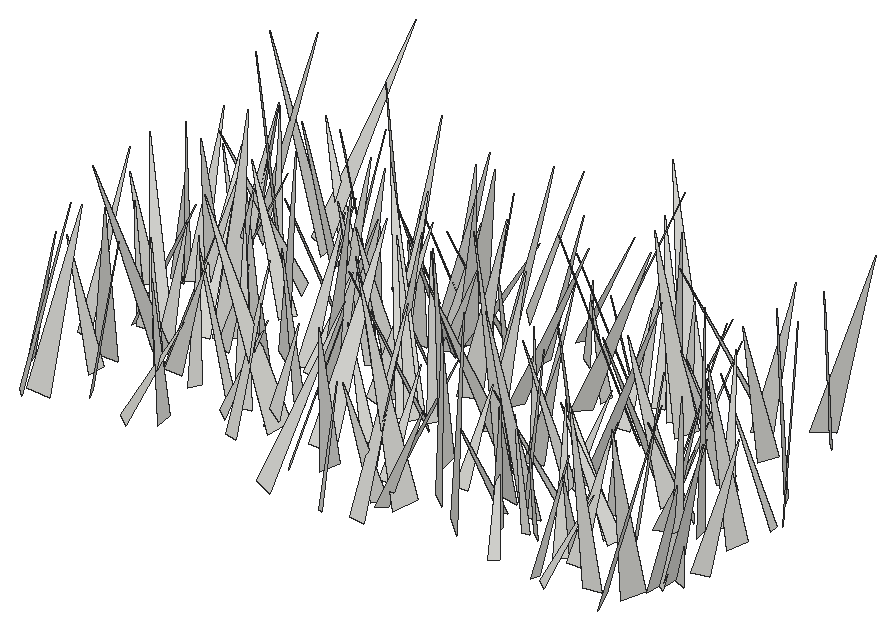
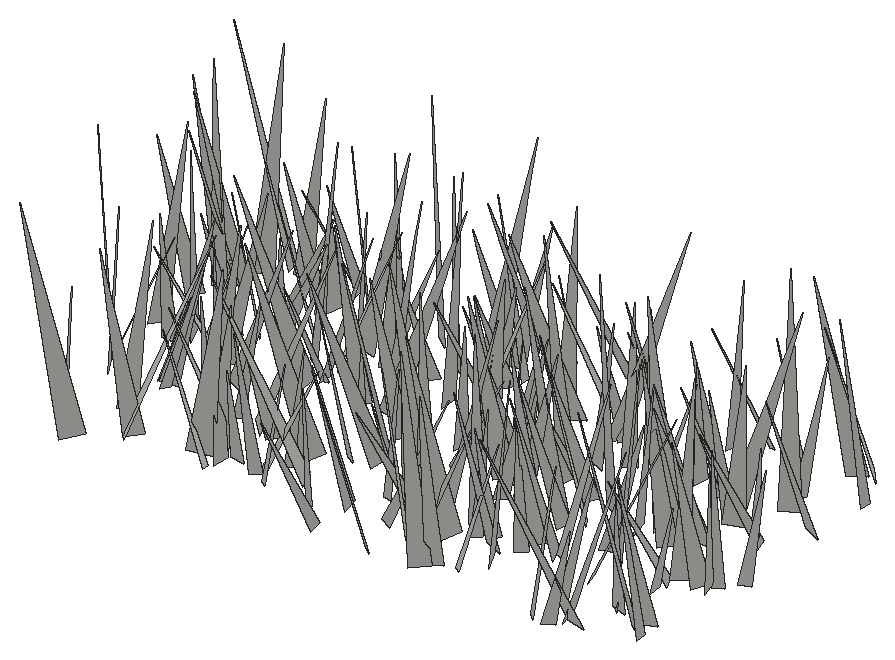
# SketchUp Ruby script. Lengths in inches.
U = 1.inch
M = Sketchup.active_model
def pt(a) = Geom::Point3d.new(a.map { |v| v * U })
def face(e, loops, mat)
  f = e.add_face(loops[0].map { |a| pt(a) })
  loops[1..].each { |l| e.add_face(l.map { |a| pt(a) }).erase! }
  f.material = f.back_material = mat if mat
  f
end
# faces: each face lists its corners as indices into pts; further lists are holes
def faces(e, pts, list, mat = nil) = list.each { |f| face(e, (f[0].is_a?(Array) ? f : [f]).map { |l| l.map { |i| pts[i] } }, mat) }
# xy, xz, yz: faces in a plane at the given z, y or x. An outline is a flat list of corners, or four numbers for a rectangle; further outlines are holes
def ring(l) = l.size == 4 ? [[l[0], l[1]], [l[2], l[1]], [l[2], l[3]], [l[0], l[3]]] : l.each_slice(2).to_a
def flat(e, list, mat, &to3) = list.each { |f| face(e, (f[0].is_a?(Array) ? f : [f]).map { |l| ring(l).map { |u, v| to3.(u, v) } }, mat) }
def xy(e, z, list, mat = nil) = flat(e, list, mat) { |x, y| [x, y, z] }
def xz(e, y, list, mat = nil) = flat(e, list, mat) { |x, z| [x, y, z] }
def yz(e, x, list, mat = nil) = flat(e, list, mat) { |y, z| [x, y, z] }
def lines(e, pts, list) = list.each { |a, b| e.add_line(pt(pts[a]), pt(pts[b])) }
# prism: a flat outline (further loops are holes) pulled along v
def prism(e, loops, v, mat = nil)
  f = face(e, loops, mat); d = Geom::Vector3d.new(v.map { |x| x * U })
  f.pushpull(f.normal.samedirection?(d) ? d.length : -d.length)
end
def box(e, o, s, mat = nil) = prism(e, [[o, [o[0] + s[0], o[1], o[2]], [o[0] + s[0], o[1] + s[1], o[2]], [o[0], o[1] + s[1], o[2]]]], [0, 0, s[2]], mat)
def at(x, y, z, deg = 0) = Geom::Transformation.translation(pt([x, y, z])) * Geom::Transformation.rotation(ORIGIN, Z_AXIS, deg.degrees)
def axes(o, x, y, z) = Geom::Transformation.new([*x, 0, *y, 0, *z, 0, *pt(o).to_a, 1])
def part(name) = M.definitions.add(name)
# library, detail: a bought-in or finely detailed component or shape, given as its bounding box
def library(name, o, s) = part(name).tap { |d| box(d.entities, o, s) }
def detail(e, o, s) = box(e.add_group.entities, o, s)
def put(e, d, t, mat = nil) = e.add_instance(d, t).tap { |i| i.material = mat if mat }
def group(e, t, mat = nil) = e.add_group.tap { |g| g.transformation = t; g.material = mat if mat }.entities
root = M.entities
c1 = part("fur_instance\#9")
p = [[0.8125,0,1.79],[0.67,-0.02,1.48],[0,-0.11,0],[0,0.11,0]]
faces(c1.entities,p,[[0,1,2,3]])
put(root,c1,axes([502.27,435.3,-21.66],[-0.87926,6.56228,2.62812],[6.83144,1.46959,-1.38397],[1.81713,-2.34956,6.47466]))
put(root,c1,axes([525.14,434.54,-21.66],[2.28996,3.33239,0.84649],[3.03653,-2.43723,1.38011],[-1.61271,0.14282,3.80053]))
put(root,c1,axes([546.94,438.2,-21.66],[6.05759,-4.04132,1.47541],[-3.82561,-6.22554,-1.34569],[-1.96821,-0.33746,7.15653]))
put(root,c1,axes([545.92,436.44,-21.66],[7.78659,2.72532,1.24866],[2.87625,-7.77148,-0.97412],[-0.84485,-1.33952,8.19204]))
put(root,c1,axes([508.52,435.88,-21.66],[2.58495,3.56171,0.23056],[3.43761,-2.40789,-1.34382],[0.96012,-0.96809,4.1907]))
put(root,c1,axes([527.24,437.77,-21.66],[2.70621,-3.86796,1.26709],[-3.69816,-2.97221,-1.17466],[-1.70008,0.30833,4.57219]))
put(root,c1,axes([510.52,437.41,-21.66],[5.22033,-0.21574,2.13038],[0.1303,-5.5713,-0.88347],[-2.13731,-0.86658,5.14955]))
put(root,c1,axes([501.4,434.64,-21.66],[4.49985,4.45709,1.03745],[4.28289,-4.6143,1.2473],[-1.61209,0.1822,6.20956]))
put(root,c1,axes([541.65,435.8,-21.66],[1.90499,3.12749,0.05078],[3.06447,-1.8542,-0.76405],[0.62675,-0.43991,3.5814]))
put(root,c1,axes([520.53,434.68,-21.66],[1.99959,6.47326,0.24716],[6.43471,-1.95494,-0.85747],[0.74746,-0.48749,6.72058]))
put(root,c1,axes([544.51,437.19,-21.66],[-0.07394,-6.12578,2.47714],[-6.56947,-0.19789,-0.68546],[-0.70961,2.47033,6.08776]))
put(root,c1,axes([499.51,437.95,-21.66],[5.83398,1.13984,1.03884],[1.35175,-5.73614,-1.2974],[-0.74243,-1.48703,5.80098]))
put(root,c1,axes([527.8,437.32,-21.66],[3.87779,-2.1954,0.31482],[-2.2129,-3.78759,0.8446],[0.14815,0.88911,4.37535]))
put(root,c1,axes([540.71,436.34,-21.66],[4.041,0.55824,1.1889],[0.26805,-4.11576,1.02147],[-1.28579,0.89645,3.94942]))
put(root,c1,axes([532.84,438.14,-21.66],[-4.52397,-6.09316,3.51067],[-6.34353,5.33763,1.08955],[3.03497,2.07386,7.51038]))
put(root,c1,axes([522.19,439.15,-21.66],[5.38586,-3.00561,1.16634],[-2.8404,-5.49795,-1.05176],[-1.52519,-0.37466,6.07741]))
put(root,c1,axes([528.85,438.31,-21.66],[-7.80525,1.8691,2.4402],[2.24771,8.01322,1.05174],[2.09664,-1.63243,7.95672]))
put(root,c1,axes([537.33,436.47,-21.66],[-3.18847,2.06393,0.29466],[1.98964,3.17316,-0.69666],[0.62286,0.42918,3.73374]))
put(root,c1,axes([527.66,435.03,-21.66],[1.84381,6.83005,0.32521],[6.75707,-1.87158,0.99709],[-1.04756,-0.05069,7.00393]))
put(root,c1,axes([525.7,438.75,-21.66],[5.69454,1.71793,1.14191],[1.95584,-5.5622,-1.38552],[-0.6557,-1.67144,5.78441]))
put(root,c1,axes([535.42,439.12,-21.66],[5.69502,0.05498,1.49404],[0.36012,-5.7612,-1.16071],[-1.45103,-1.21405,5.57575]))
put(root,c1,axes([504.93,437.25,-21.66],[4.32331,2.64676,1.47041],[2.57631,-4.56233,0.63737],[-1.59061,-0.19566,5.02892]))
put(root,c1,axes([540.91,440.02,-21.66],[3.64038,-1.44849,0.64201],[-1.22649,-3.59476,-1.15586],[-1.003,-0.8615,3.74359]))
put(root,c1,axes([503.36,439.67,-21.66],[-4.62696,1.13691,1.70574],[1.48296,4.76376,0.84751],[1.41525,-1.27471,4.68861]))
put(root,c1,axes([502.73,441.37,-21.66],[1.80193,-7.44469,0.50754],[-7.36471,-1.69029,1.35351],[1.20089,0.80465,7.53912]))
put(root,c1,axes([520.26,437.6,-21.66],[4.1336,3.03674,0.5342],[2.87698,-4.11997,1.15876],[-1.10914,0.6308,4.99657]))
put(root,c1,axes([541.75,438.98,-21.66],[-1.54169,4.36128,2.00643],[4.43238,2.10262,-1.16464],[1.84406,-1.40768,4.47674]))
put(root,c1,axes([537.59,440.31,-21.66],[-1.86728,-3.21645,1.13397],[-3.16749,2.11482,0.78275],[1.26429,0.54787,3.63587]))
put(root,c1,axes([530.01,440.18,-21.66],[-3.26006,-5.04679,2.60885],[-5.29814,3.78652,0.70434],[2.05082,1.75965,5.96674]))
put(root,c1,axes([547.6875,441.08,-21.66],[6.64533,-1.36705,0.39109],[-1.31179,-6.61549,-0.83466],[-0.54862,-0.74069,6.73295]))
put(root,c1,axes([534.12,441.43,-21.66],[-0.56318,-3.80765,0.20803],[-3.75255,0.51599,-0.71463],[-0.67806,0.30692,3.78215]))
put(root,c1,axes([515.02,438.35,-21.66],[1.99951,5.4557,0.6063],[5.41529,-2.06607,0.73224],[-0.89823,-0.31139,5.76424]))
put(root,c1,axes([516.68,441.11,-21.66],[-8.04315,1.60644,1.39343],[1.83623,7.99603,1.38066],[1.07265,-1.64234,8.08496]))
put(root,c1,axes([547.78,441.375,-21.66],[-1.4348,-7.0433,2.45033],[-7.23254,1.92235,1.29061],[1.81726,2.08982,7.07114]))
put(root,c1,axes([512.89,440.21,-21.66],[2.48404,3.35431,0.63876],[3.34518,-2.23213,-1.28736],[0.685,-1.26336,3.97047]))
put(root,c1,axes([527.1,439.61,-21.66],[-1.4583,4.1794,0.64732],[4.14586,1.27741,1.09233],[-0.83566,-0.95598,4.28962]))
put(root,c1,axes([540.46,439.14,-21.66],[-4.55116,2.07867,0.64916],[1.93391,4.54938,-1.00919],[1.00113,0.66152,4.90056]))
put(root,c1,axes([547.33,439.67,-21.66],[6.67173,1.075,1.66778],[0.88806,-6.84957,0.86244],[-1.77439,0.61387,6.70252]))
put(root,c1,axes([536.15,440.92,-21.66],[-4.08433,-4.26667,3.28401],[-4.58243,4.91876,0.69141],[2.82675,1.80893,5.86585]))
put(root,c1,axes([536.89,440.19,-21.66],[0.66208,3.60921,1.19442],[3.54519,-1.02396,1.12897],[-1.37285,-0.90361,3.49144]))
put(root,c1,axes([533.46,442.82,-21.66],[0.2783,-5.0487,0.14304],[-4.93686,-0.24166,1.07529],[1.0664,0.19877,4.94071]))
put(root,c1,axes([547.35,440.32,-21.66],[2.91311,4.64162,1.0633],[4.76072,-2.81168,-0.76908],[0.10392,-1.30816,5.4258]))
put(root,c1,axes([516.2,440.87,-21.66],[-1.839,3.01934,1.93742],[3.07994,2.44517,-0.88715],[1.83955,-1.07548,3.42218]))
put(root,c1,axes([526.01,439.94,-21.66],[-2.24412,3.20659,0.81725],[3.00578,2.38826,-1.11699],[1.38398,0.01256,3.75108]))
put(root,c1,axes([535.91,441.9375,-21.66],[-0.62718,-6.98929,2.39617],[-7.29856,0.2117,-1.29283],[-1.15016,2.46782,6.89725]))
put(root,c1,axes([513.98,443.21,-21.66],[1.58205,-4.94043,0.08132],[-4.90313,-1.55912,0.66773],[0.6114,0.28046,5.1444]))
put(root,c1,axes([507.17,442.52,-21.66],[2.31038,-4.41979,0.71264],[-4.3801,-2.06578,1.38834],[0.92579,1.25629,4.79008]))
put(root,c1,axes([505.16,443.98,-21.66],[-0.75565,-7.24529,1.23648],[-7.25287,0.53359,-1.30585],[-1.19119,1.34729,7.16659]))
put(root,c1,axes([541.84,442.8,-21.66],[-4.37284,2.10544,0.41102],[2.13916,4.20984,1.19366],[-0.16073,-1.25217,4.70423]))
put(root,c1,axes([513.35,441.64,-21.66],[-0.65155,5.99766,1.58433],[6.18323,0.49957,0.65163],[-0.49968,-1.63861,5.99765]))
put(root,c1,axes([509.35,441.95,-21.66],[-4.59387,1.36569,1.34916],[1.20913,4.77619,-0.71765],[1.49109,0.33451,4.73854]))
put(root,c1,axes([535.74,444.74,-21.66],[-3.80651,-3.12707,0.03174],[-3.06593,3.74155,0.93273],[0.61617,-0.70095,4.83716]))
put(root,c1,axes([538.64,443.25,-21.66],[3.81482,2.67004,0.71919],[2.75746,-3.58156,-1.32965],[0.20681,-1.49748,4.4625]))
put(root,c1,axes([530.23,442.125,-21.66],[-1.29453,3.3269,0.92168],[3.25121,1.50588,-0.8692],[1.16077,-0.50757,3.46245]))
put(root,c1,axes([548.49,442.92,-21.66],[3.34726,-4.07819,1.53745],[-4.35777,-3.09938,1.26621],[0.07255,1.99042,5.12177]))
put(root,c1,axes([520.33,440.74,-21.66],[-1.86477,7.56726,1.18834],[7.49142,2.05683,-1.34204],[1.5982,-0.81177,7.67722]))
put(root,c1,axes([511.8,442.32,-21.66],[-4.83845,-0.36416,0.05457],[-0.36621,4.6838,-1.21411],[-0.03844,1.21473,4.69778]))
put(root,c1,axes([527.66,443.93,-21.66],[-7.27615,-1.41209,3.18772],[-1.2687,7.94356,0.62294],[3.24745,-0.06052,7.38568]))
put(root,c1,axes([505.96,442.62,-21.66],[0.1057,3.9764,0.92499],[3.9126,-0.36287,1.11284],[-1.16573,-0.85739,3.81897]))
put(root,c1,axes([541.29,443.12,-21.66],[-3.62089,2.64212,0.01483],[2.58278,3.53416,0.96476],[-0.55698,-0.78788,4.37731]))
put(root,c1,axes([522.07,443.17,-21.66],[-2.23276,3.13779,0.67741],[3.20125,2.1153,0.75324],[-0.23799,-0.9847,3.77672]))
put(root,c1,axes([537.34,445.16,-21.66],[-4.05006,-5.82532,2.03849],[-5.82326,4.4146,1.04584],[2.04438,1.03428,7.01738]))
put(root,c1,axes([525.23,442.81,-21.66],[4.11341,0.99659,0.14821],[0.94897,-4.04143,0.83763],[-0.33855,0.78037,4.1487]))
put(root,c1,axes([506.24,442.92,-21.66],[4.19181,1.99584,0.5753],[1.88629,-4.2003,0.82769],[-0.86965,0.50967,4.56832]))
put(root,c1,axes([515.68,444.32,-21.66],[-1.40726,-4.75955,2.034],[-5.17479,1.24906,-0.65748],[-0.10975,2.13481,4.91949]))
put(root,c1,axes([539.56,445.42,-21.66],[0.99148,-3.49866,0.36174],[-3.47594,-0.91715,0.65665],[0.53788,0.52224,3.57665]))
put(root,c1,axes([523.57,447.09,-21.66],[-4.47092,-4.93614,0.16266],[-4.90041,4.46105,0.68268],[0.61475,-0.33851,6.62484]))
put(root,c1,axes([504.69,444.75,-21.66],[-2.17172,3.54056,2.13295],[3.72846,2.71807,-0.7156],[1.78427,-1.37037,4.09143]))
put(root,c1,axes([529.65,447.36,-21.66],[0.11863,-7.1905,0.64579],[-7.08435,-0.24031,-1.37429],[-1.39009,0.61104,7.05894]))
put(root,c1,axes([499.92,442.72,-21.66],[1.80185,5.93958,0.37976],[5.89361,-1.83593,0.75111],[-0.82954,-0.14229,6.16126]))
put(root,c1,axes([522,444.73,-21.66],[-3.20539,-1.99252,1.2784],[-2.28309,3.17085,-0.78241],[0.62603,1.36182,3.69222]))
put(root,c1,axes([543.06,445.69,-21.66],[3.00481,-2.76961,0.12717],[-2.71494,-2.90128,0.96303],[0.56213,0.79222,3.97142]))
put(root,c1,axes([542.36,444.25,-21.66],[3.86177,3.77021,1.4507],[3.73701,-4.09632,0.69796],[-1.5342,-0.48777,5.35169]))
put(root,c1,axes([535.49,446.4,-21.66],[-5.30182,-0.75056,0.88287],[-0.65483,5.35184,0.61739],[0.95603,-0.49663,5.31898]))
put(root,c1,axes([531.5,444.85,-21.66],[-7.85501,-1.13743,1.66782],[-1.3997,7.89692,-1.20666],[1.45472,1.45652,7.84468]))
put(root,c1,axes([504.36,444.9,-21.66],[-3.46559,5.8146,1.30946],[5.95968,3.40104,0.67057],[0.08042,-1.46897,6.73574]))
put(root,c1,axes([548.03,447.12,-21.66],[-6.01027,1.97565,2.91231],[2.62602,6.35479,1.10849],[2.3428,-2.05464,6.22879]))
put(root,c1,axes([515.82,446.94,-21.66],[7.89082,-0.9052,1.78608],[-0.78265,-8.07818,-0.63641],[-1.84308,-0.44515,7.91703]))
put(root,c1,axes([531.8,447.35,-21.66],[3.60736,-4.41491,0.21347],[-4.38405,-3.53869,0.89879],[0.56311,0.73233,5.62998]))
put(root,c1,axes([502.08,445.66,-21.66],[0.5553,3.90242,1.15183],[3.90207,-0.84018,0.96535],[-1.15302,-0.96393,3.8217]))
put(root,c1,axes([507.74,446.6875,-21.66],[1.20072,-3.47995,0.99765],[-3.52529,-0.88496,1.15597],[0.82322,1.28603,3.49507]))
put(root,c1,axes([543.75,448.16,-21.66],[-3.41692,-2.65793,0.41527],[-2.50813,3.39027,1.06197],[0.9728,-0.5949,4.19669]))
put(root,c1,axes([501.49,445.875,-21.66],[4.45385,0.90104,0.34779],[0.77968,-4.32278,1.21461],[-0.57002,1.12752,4.37874]))
put(root,c1,axes([535.33,446.58,-21.66],[0.85166,3.52496,0.51911],[3.494,-0.72175,-0.83136],[0.69768,-0.68839,3.5298]))
put(root,c1,axes([511.42,448.13,-21.66],[-3.32783,-6.52848,3.29816],[-6.89122,4.01297,0.99019],[2.45153,2.41834,7.26051]))
put(root,c1,axes([541.49,448.66,-21.66],[-5.54142,2.04017,2.02802],[2.50487,5.58649,1.22443],[1.41448,-1.90035,5.77671]))
put(root,c1,axes([545.33,446.88,-21.66],[-6.71268,-1.89599,2.76742],[-2.51748,6.93875,-1.3526],[2.21714,2.13833,6.8429]))
put(root,c1,axes([507.07,447.98,-21.66],[-5.12716,5.45276,3.67809],[5.84452,5.9162,-0.62364],[3.01704,-2.19425,7.45865]))
put(root,c1,axes([535.95,447.55,-21.66],[7.40622,-0.19557,0.80001],[-0.28757,-7.3972,0.85392],[-0.77173,0.87956,7.35943]))
put(root,c1,axes([522.49,447.04,-21.66],[-5.52094,1.92393,0.48296],[1.85996,5.5174,-0.71721],[0.68943,0.52184,5.80241]))
put(root,c1,axes([519.83,448.16,-21.66],[5.84499,-0.86217,1.83487],[-1.09003,-6.05756,0.62599],[-1.70936,0.91471,5.87498]))
put(root,c1,axes([505.89,449.55,-21.66],[3.45559,-4.90486,0.92565],[-4.98413,-3.32981,0.96246],[0.2699,1.30779,5.9222]))
put(root,c1,axes([513.93,447.49,-21.66],[-0.30009,3.62925,0.24074],[3.53668,0.34756,-0.831],[0.84929,-0.16496,3.54556]))
put(root,c1,axes([523.67,447.6875,-21.66],[-5.20641,1.3754,0.94823],[1.21962,5.25029,-0.91901],[1.14166,0.66356,5.30602]))
put(root,c1,axes([522.17,447.1875,-21.66],[-4.81407,6.51041,0.79127],[6.55623,4.75265,0.78417],[-0.16528,-1.10168,8.05889]))
put(root,c1,axes([504.21,447.99,-21.66],[1.48764,5.46016,1.29529],[5.56167,-1.25605,-1.09283],[0.74757,-1.52092,5.55267]))
put(root,c1,axes([519.22,447.31,-21.66],[1.31333,6.20143,0.89],[6.24264,-1.21867,-0.72041],[0.52849,-1.01577,6.2979]))
put(root,c1,axes([539.47,450.33,-21.66],[-1.836,-5.36618,0.72675],[-5.38286,1.72484,-0.86298],[-0.59066,0.96126,5.60554]))
put(root,c1,axes([513.17,447.97,-21.66],[-3.03856,4.16793,1.35783],[3.96538,3.31773,-1.3102],[1.86846,-0.26309,4.98878]))
put(root,c1,axes([517.71,449.58,-21.66],[-1.21907,-3.82959,1.50139],[-4.09681,0.98993,-0.80143],[-0.36895,1.66143,3.93822]))
put(root,c1,axes([505.54,447.04,-21.66],[-3.21539,5.33291,0.27404],[5.21793,3.20577,-1.16191],[1.13501,0.36996,6.11789]))
put(root,c1,axes([530.96,448.41,-21.66],[-3.9297,0.38452,0.60241],[0.18265,3.7953,-1.23109],[0.69093,1.18368,3.75164]))
put(root,c1,axes([527.22,449.1,-21.66],[4.47757,-3.00826,2.16701],[-3.51648,-4.52249,0.98776],[-1.1747,2.07164,5.30307]))
put(root,c1,axes([508.57,448.99,-21.66],[-5.92753,-0.80933,1.51712],[-1.07571,5.99367,-1.00549],[1.34146,1.2301,5.89742]))
put(root,c1,axes([522.33,450.33,-21.66],[-2.45002,-3.17903,0.27674],[-3.09062,2.27713,-1.20338],[-0.79426,0.94543,3.82893]))
put(root,c1,axes([546.05,448.42,-21.66],[-0.40963,5.6712,0.85204],[5.69515,0.30195,0.72827],[-0.67361,-0.89587,5.63914]))
put(root,c1,axes([499.08,450.42,-21.66],[2.35364,-2.97334,1.61897],[-3.0072,-2.74184,-0.66374],[-1.55518,0.80187,3.73361]))
put(root,c1,axes([519.03,449.18,-21.66],[-3.21117,5.73542,2.2751],[5.803,3.67883,-1.08356],[2.09673,-1.39782,6.48325]))
put(root,c1,axes([517.64,451.3125,-21.66],[-5.01187,1.13995,1.85475],[1.60842,5.07616,1.22637],[1.46717,-1.67079,4.99142]))
put(root,c1,axes([511.62,450.35,-21.66],[5.2265,3.38981,1.10604],[3.55749,-5.09026,-1.20993],[-0.2416,-1.62138,6.11091]))
put(root,c1,axes([513.7,450.38,-21.66],[1.63751,6.97927,2.94123],[7.53115,-1.18196,-1.38823],[0.80173,-3.15202,7.03309]))
put(root,c1,axes([548.45,450.1875,-21.66],[-4.94313,-1.68267,0.02369],[-1.64372,4.81198,-1.18726],[-0.36076,1.13137,5.08492]))
put(root,c1,axes([516.32,450.87,-21.66],[0.21554,-5.31829,2.18174],[-5.56977,-0.73327,-1.23719],[-1.42193,2.0661,5.17688]))
put(root,c1,axes([500.17,451.67,-21.66],[0.87128,-4.23502,0.75689],[-4.24446,-0.72019,0.85631],[0.702,0.90186,4.23807]))
put(root,c1,axes([502.62,452.39,-21.66],[5.63565,-3.00774,1.4531],[-2.80235,-5.80815,-1.15361],[-1.81792,-0.37081,6.28301]))
put(root,c1,axes([542.6875,452.71,-21.66],[1.51534,-5.37644,0.92666],[-5.31705,-1.67082,-0.99923],[-1.22223,0.60275,5.49581]))
put(root,c1,axes([548.05,451.66,-21.66],[-5.21121,-4.35385,3.58957],[-4.50193,6.15376,0.92827],[3.40202,1.4741,6.72689]))
put(root,c1,axes([541.59,448.84,-21.66],[4.07971,3.91858,0.07723],[3.79656,-3.97882,1.32677],[-0.97331,0.90496,5.499]))
put(root,c1,axes([523.4,451.45,-21.66],[4.4224,-5.22883,1.99199],[-5.58659,-4.26873,1.19762],[-0.31423,2.30295,6.7427]))
put(root,c1,axes([512.45,451.54,-21.66],[4.92372,-1.23429,0.65682],[-1.32256,-4.89156,0.72207],[-0.45359,0.86432,5.02445]))
put(root,c1,axes([536.63,453.43,-21.66],[3.04717,-2.22298,0.43436],[-2.028,-3.00193,-1.13631],[-1.00873,-0.67996,3.59662]))
put(root,c1,axes([542.6,453.26,-21.66],[-4.67386,-0.0885,1.27111],[0.2568,4.66814,1.26925],[1.24804,-1.29194,4.49909]))
put(root,c1,axes([510.14,454.72,-21.66],[-2.61623,-5.06997,0.16776],[-4.93297,2.58676,1.24576],[1.18261,-0.42604,5.56752]))
put(root,c1,axes([508.39,452.31,-21.66],[-3.73959,3.61146,1.09906],[3.77498,3.58144,1.07604],[0.00944,-1.53809,5.08619]))
put(root,c1,axes([543.7,452.37,-21.66],[-3.57996,-1.2077,0.30439],[-1.24532,3.48547,-0.8173],[0.0195,0.87192,3.68872]))
put(root,c1,axes([534.96,453.65,-21.66],[-5.01465,-5.39389,0.78065],[-5.43536,4.87162,-1.25473],[-0.40033,1.42249,7.25716]))
put(root,c1,axes([518.89,455.26,-21.66],[-2.89154,-5.8907,0.51675],[-5.81601,2.937,0.93617],[1.06836,0.04534,6.49499]))
put(root,c1,axes([526.29,452.44,-21.66],[6.61677,-1.08212,0.53072],[-1.15649,-6.53431,1.0953],[-0.3394,1.16883,6.6146]))
put(root,c1,axes([500.52,452.15,-21.66],[-4.80095,-0.85986,1.55653],[-1.24807,4.82151,-1.18603],[1.26668,1.49164,4.73094]))
put(root,c1,axes([516.71,454.69,-21.66],[1.30695,-5.86281,0.96642],[-5.89292,-1.15208,0.98022],[0.76158,1.14664,5.9262]))
put(root,c1,axes([528.02,453.21,-21.66],[2.95558,3.83246,1.3061],[4.0436,-2.87668,-0.7093],[-0.20723,-1.47175,4.78749]))
put(root,c1,axes([501.09,452.22,-21.66],[-4.2045,3.84796,1.64776],[3.68267,4.51063,-1.13666],[1.98995,-0.21727,5.58504]))
put(root,c1,axes([512.33,454.33,-21.66],[4.00541,-4.88826,1.49079],[-5.10449,-3.91872,0.86522],[-0.24835,1.7057,6.26017]))
put(root,c1,axes([546.9,453.42,-21.66],[-5.34444,-2.84039,2.21318],[-3.30562,5.4408,-0.99979],[1.42788,1.96442,5.96919]))
put(root,c1,axes([506.96,455.75,-21.66],[-5.82237,-2.50943,0.01956],[-2.48564,5.77362,0.82736],[0.34528,-0.75212,6.28591]))
put(root,c1,axes([529.86,454.46,-21.66],[6.60673,-3.01857,0.44503],[-3.04917,-6.49303,1.22551],[0.11127,1.29906,7.15953]))
put(root,c1,axes([503.01,452.99,-21.66],[4.04294,1.47662,0.10602],[1.40514,-3.92456,1.07725],[-0.46609,0.97696,4.16717]))
put(root,c1,axes([512.49,455.69,-21.66],[1.67883,-4.20753,0.33675],[-4.18563,-1.61266,0.71764],[0.54516,0.57551,4.47289]))
put(root,c1,axes([519.27,456.4,-21.66],[6.44633,-3.37101,0.63256],[-3.2949,-6.46051,-0.8512],[-0.95262,-0.46602,7.22457]))
put(root,c1,axes([523.14,455.65,-21.66],[-1.38247,-3.90181,0.99129],[-3.91317,1.54858,0.63797],[0.94545,0.70412,4.09003]))
put(root,c1,axes([518.7,455.1,-21.66],[3.23817,-2.36152,0.30304],[-2.37388,-3.16317,0.7165],[0.18248,0.75624,3.94324]))
put(root,c1,axes([515.875,455.92,-21.66],[3.30583,-2.31707,0.74955],[-2.21165,-3.38553,-0.71128],[-1.01942,-0.16893,3.97384]))
put(root,c1,axes([524.41,453.36,-21.66],[1.50713,3.43781,0.3216],[3.3001,-1.53741,0.96906],[-1.01552,0.10596,3.62641]))
put(root,c1,axes([523.75,453.92,-21.66],[-3.45696,-5.56122,4.74392],[-6.59951,4.63089,0.61955],[3.14299,3.60698,6.51874]))
put(root,c1,axes([542.74,456.83,-21.66],[4.44508,-4.04211,0.97735],[-3.87336,-4.54492,-1.18043],[-1.51359,-0.24009,5.89101]))
put(root,c1,axes([538.5,453.52,-21.66],[3.62249,2.81644,0.55831],[2.6251,-3.61284,1.19278],[-1.16313,0.61769,4.43081]))
put(root,c1,axes([502.98,454.39,-21.66],[-4.26519,0.30143,0.24037],[0.24291,4.17451,-0.92459],[0.29939,0.9072,4.17466]))
put(root,c1,axes([533.35,454.15,-21.66],[-1.89071,3.52857,0.74513],[3.44423,2.01617,-0.80816],[1.06925,-0.25501,3.92077]))
put(root,c1,axes([536.8,456.16,-21.66],[-6.28621,2.90163,2.83322],[3.4688,6.55463,0.9835],[2.10096,-2.14018,6.85337]))
put(root,c1,axes([514.8,455.37,-21.66],[2.68991,-2.47286,1.2383],[-2.72716,-2.65872,0.6147],[-0.45937,1.30393,3.60178]))
put(root,c1,axes([530.28,456.39,-21.66],[3.55115,-1.15094,1.45453],[-0.93925,-3.82501,-0.73353],[-1.59941,-0.30919,3.66022]))
put(root,c1,axes([520.47,456.74,-21.66],[1.50872,-3.69838,0.31644],[-3.67115,-1.43625,0.71715],[0.54852,0.55997,3.92937]))
put(root,c1,axes([510.64,454.62,-21.66],[5.6278,2.51424,1.57514],[2.22036,-5.80941,1.3399],[-1.96786,0.63554,6.01649]))
put(root,c1,axes([517.78,456.24,-21.66],[-0.77592,-4.15559,2.31409],[-4.39268,1.52537,1.26634],[1.82437,1.90534,4.03328]))
put(root,c1,axes([503.63,457.55,-21.66],[-5.15951,-5.90719,2.53837],[-5.9684,5.61072,0.92562],[2.3909,1.25844,7.78837]))
put(root,c1,axes([521.29,458.07,-21.66],[-1.6318,-4.41068,0.10105],[-4.3461,1.58854,-0.8456],[-0.75876,0.38671,4.62621]))
put(root,c1,axes([535.83,457.16,-21.66],[0.28341,4.29415,2.46111],[4.89058,0.13603,-0.80051],[0.76092,-2.47364,4.22839]))
put(root,c1,axes([540.94,459.52,-21.66],[-5.31992,-4.92486,0.01845],[-4.88394,5.27914,0.91325],[0.63384,-0.65774,7.19179]))
put(root,c1,axes([518.76,457.74,-21.66],[-2.91318,-3.12111,0.33199],[-3.12229,2.8354,-0.74159],[-0.32068,0.74655,4.20452]))
put(root,c1,axes([517.14,456.83,-21.66],[6.46627,-2.11143,1.67342],[-2.36842,-6.52888,0.91405],[-1.28416,1.40953,6.74057]))
put(root,c1,axes([534.05,458.4,-21.66],[6.7511,0.38921,2.10678],[0.68602,-6.99103,-0.90679],[-2.02963,-1.06837,6.70124]))
put(root,c1,axes([519.35,456.62,-21.66],[4.38555,-0.36882,0.03632],[-0.36139,-4.16033,1.38975],[0.08213,1.3878,4.17584]))
put(root,c1,axes([530.29,458.91,-21.66],[-2.2334,-3.12116,0.78897],[-3.02774,2.36275,0.77617],[1.09405,0.16724,3.75863]))
put(root,c1,axes([531.11,457.99,-21.66],[-3.78552,-3.06993,0.30173],[-3.01727,3.58565,-1.37288],[-0.64154,1.25071,4.67652]))
put(root,c1,axes([531.41,458.27,-21.66],[-0.36242,4.3186,2.109],[4.6668,0.82166,-0.88056],[1.14855,-1.97588,4.24338]))
put(root,c1,axes([514.19,459.89,-21.66],[-2.66612,-3.28273,0.28859],[-3.19335,2.6653,0.81637],[0.81369,-0.29607,4.14946]))
put(root,c1,axes([514.14,456.39,-21.66],[2.11808,6.39246,0.96016],[6.39192,-2.22182,0.69185],[-0.96378,-0.68681,6.6986]))
put(root,c1,axes([519.23,458.6,-21.66],[4.62058,2.87983,1.50344],[3.15499,-4.60106,-0.88304],[-0.77446,-1.56215,5.37246]))
put(root,c1,axes([535.46,457.06,-21.66],[-3.34888,5.66427,0.75226],[5.70524,3.26636,0.80369],[-0.31635,-1.05439,6.53093]))
put(root,c1,axes([513.25,457.67,-21.66],[-6.49961,-2.89491,2.26898],[-3.37847,6.5202,-1.35892],[1.4542,2.20912,6.98418]))
put(root,c1,axes([500.46,457.95,-21.66],[0.08637,4.97569,1.67082],[5.15736,0.22998,-0.95146],[0.97504,-1.65717,4.88463]))
put(root,c1,axes([528.58,456.84,-21.66],[7.17048,3.0592,0.30714],[3.02615,-7.16002,0.66735],[-0.54355,0.49421,7.76718]))
put(root,c1,axes([526.38,459.29,-21.66],[-1.07299,-3.39329,1.1863],[-3.30809,1.41653,1.05972],[1.4065,0.74301,3.39746]))
put(root,c1,axes([524.35,457.8125,-21.66],[5.06172,0.87175,1.3003],[0.68802,-5.19178,0.80241],[-1.40619,0.59773,5.07318]))
put(root,c1,axes([503.1875,457.71,-21.66],[0.59003,4.76484,1.13067],[4.77949,-0.80843,0.91275],[-1.06703,-0.9864,4.71367]))
put(root,c1,axes([540.37,459.14,-21.66],[-2.5167,4.57974,3.46384],[4.9953,3.61127,-1.14527],[2.83182,-2.30014,5.09864]))
put(root,c1,axes([500,459.51,-21.66],[5.07227,1.20948,1.05659],[1.39553,-5.05165,-0.91676],[-0.7948,-1.15114,5.13326]))
put(root,c1,axes([534.41,459.54,-21.66],[4.26627,1.55205,0.05399],[1.49304,-4.05567,-1.39111],[0.42732,-1.32496,4.32143]))
put(root,c1,axes([533.4,457.62,-21.66],[-0.37252,4.33667,0.3989],[4.3129,0.31185,0.63743],[-0.60398,-0.44793,4.30572]))
put(root,c1,axes([506.41,459.32,-21.66],[-1.858,-4.3991,1.45242],[-4.62148,1.65138,-0.9103],[-0.32175,1.68364,4.68782]))
put(root,c1,axes([516.2,461.05,-21.66],[4.17782,-5.39394,0.17375],[-5.37681,-4.14138,0.71959],[0.46328,0.57738,6.78461]))
put(root,c1,axes([535.73,458.35,-21.66],[-3.99948,7.12267,1.32626],[7.23474,3.8453,1.16596],[-0.38726,-1.72292,8.0851]))
put(root,c1,axes([500.69,459.11,-21.66],[4.61104,6.12434,1.67223],[6.3457,-4.50796,-0.9879],[-0.18966,-1.93296,7.60219]))
put(root,c1,axes([515.64,460.39,-21.66],[2.0151,-5.02328,1.60572],[-5.27188,-1.87389,0.75376],[0.13771,1.76848,5.35965]))
put(root,c1,axes([505.15,460.2,-21.66],[-7.20158,-1.52489,0.67202],[-1.60184,7.15641,-0.92717],[0.45935,1.04894,7.30263]))
put(root,c1,axes([506.88,461.71,-21.66],[-3.29784,-3.61715,1.25797],[-3.53735,3.51322,0.8285],[1.46745,0.33986,4.82422]))
put(root,c1,axes([544.67,460.56,-21.66],[-3.59286,-3.26733,2.03566],[-3.70516,3.69058,-0.61592],[1.04455,1.85261,4.81713]))
put(root,c1,axes([543.1875,461.68,-21.66],[6.11915,-4.70581,1.11272],[-4.83462,-5.98952,1.25659],[-0.09634,1.67568,7.61641]))
put(root,c1,axes([519.98,461.52,-21.66],[4.42305,4.26534,0.99754],[4.37397,-4.22348,-1.33498],[0.23791,-1.64944,5.99786]))
put(root,c1,axes([505.51,461.77,-21.66],[-2.80157,3.07223,0.58027],[3.12461,2.72376,0.66487],[-0.11008,-0.87559,4.10431]))
put(root,c1,axes([524.36,461.21,-21.66],[4.0884,0.15219,0.34801],[0.0557,-3.96154,1.07814],[-0.37573,1.0688,3.94662]))
put(root,c1,axes([504.14,460.77,-21.66],[2.50136,7.65725,0.1478],[7.63522,-2.48107,-0.67805],[0.59891,-0.35058,8.02686]))
